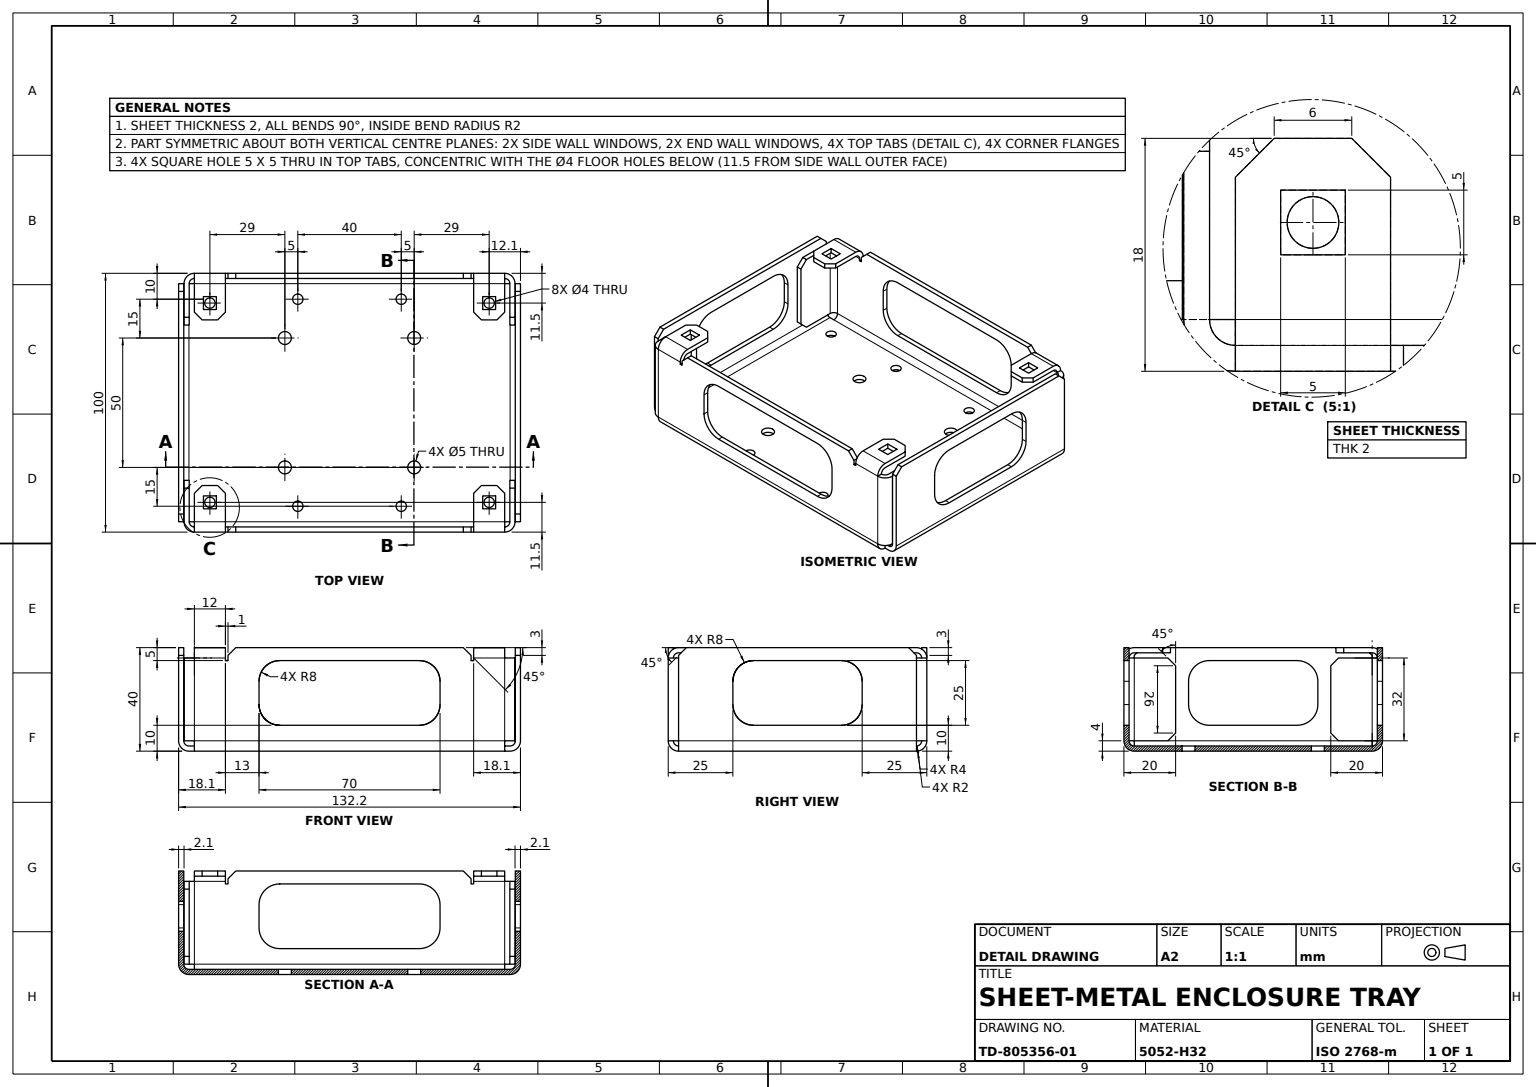
solid
v1 (51.5,38,-36)
v2 (56.5,38,-36)
e1 v1 v2 LINE
v3 (51.5,40,-36)
e2 v1 v3 LINE
v4 (56.5,40,-36)
e3 v3 v4 LINE
e4 v2 v4 LINE
face PLANE(AX(P(51.5,38,-36),D(0,0,1),D(0,-1,0))) rev [-e1 e2 e3 -e4]
v5 (54,0,36.5)
v6 (54,2,36.5)
e5 v5 v6 LINE
v7 (54,0,40.5)
e6 v5 v7 CIRCLE(AX(P(54,0,38.5),D(0,-1,0),D(0,0,-1)),2)
v8 (54,2,40.5)
e7 v7 v8 LINE
e8 v8 v6 CIRCLE(AX(P(54,2,38.5),D(0,1,0),D(0,0,1)),2)
face CYL(AX(P(54,-8,38.5),D(0,1,0),D(0,0,1)),2) rev [-e5 e6 e7 e8]
v9 (62,4,46)
v10 (64,4,46)
e9 v9 v10 LINE
v11 (60,4,50)
e10 v10 v11 CIRCLE(AX(P(60,4,46),D(0,-1,0),D(0,0,-1)),4)
v12 (60,4,48)
e11 v12 v11 LINE
e12 v9 v12 CIRCLE(AX(P(60,4,46),D(0,-1,0),D(0,0,-1)),2)
face PLANE(AX(P(60,4,46),D(0,1,0),D(0,0,1))) rev [e9 e10 -e11 -e12]
v13 (62.1,0,46)
v14 (60,0,46)
e13 v13 v14 LINE
v15 (62.1,2,46)
e14 v15 v13 LINE
v16 (60,2,46)
e15 v15 v16 LINE
e16 v16 v14 LINE
face PLANE(AX(P(62.1,2,46),D(0,0,-1),D(0,-1,0))) rev [-e13 -e14 e15 e16]
v17 (-62,4,46)
v18 (-62,36,46)
e17 v17 v18 LINE
v19 (-60,36,48)
e18 v18 v19 CIRCLE(AX(P(-60,36,46),D(0,1,0),D(0,0,1)),2)
v20 (-60,4,48)
e19 v20 v19 LINE
e20 v20 v17 CIRCLE(AX(P(-60,4,46),D(0,-1,0),D(0,0,1)),2)
face CYL(AX(P(-60,36,46),D(0,1,0),D(-1,0,0)),2) rev [e17 e18 -e19 e20]
v21 (-51,40,-32)
v22 (-48,40,-35)
e21 v21 v22 LINE
v23 (-51,38,-32)
e22 v23 v21 LINE
v24 (-48,38,-35)
e23 v24 v23 LINE
e24 v22 v24 LINE
face PLANE(AX(P(-48,40,-35),D(-0.707106781,0,-0.707106781),D(0,-1,0))) rev [-e21 -e22 -e23 -e24]
v25 (60,40,35)
v26 (57,40,32)
e25 v25 v26 LINE
v27 (60,38,35)
e26 v27 v25 LINE
v28 (57,38,32)
e27 v28 v27 LINE
e28 v26 v28 LINE
face PLANE(AX(P(57,40,32),D(-0.707106781,0,0.707106781),D(0,-1,0))) rev [-e25 -e26 -e27 -e28]
v29 (62.1,0,-46)
v30 (60,0,-46)
e29 v29 v30 LINE
v31 (60,2,-46)
e30 v31 v30 LINE
v32 (62.1,2,-46)
e31 v32 v31 LINE
e32 v32 v29 LINE
face PLANE(AX(P(62.1,2,-46),D(0,0,-1),D(0,-1,0))) [e29 -e30 -e31 e32]
v33 (-56.5,40,-36)
v34 (-51.5,40,-36)
e33 v33 v34 LINE
v35 (-51.5,38,-36)
e34 v35 v34 LINE
v36 (-56.5,38,-36)
e35 v36 v35 LINE
e36 v36 v33 LINE
face PLANE(AX(P(-51.5,38,-36),D(0,0,1),D(0,-1,0))) rev [e33 -e34 -e35 e36]
v37 (47,37,50)
v38 (44,40,50)
e37 v37 v38 LINE
v39 (47,37,48)
e38 v39 v37 LINE
v40 (44,40,48)
e39 v40 v39 LINE
e40 v38 v40 LINE
face PLANE(AX(P(47,37,48),D(-0.707106781,-0.707106781,0),D(0,0,1))) rev [-e37 -e38 -e39 -e40]
v41 (62,4,33)
e41 v9 v41 LINE
v42 (64,4,33)
e42 v41 v42 LINE
e43 v10 v42 LINE
face PLANE(AX(P(64,4,30),D(0,1,0),D(0,0,1))) rev [-e9 e41 e42 -e43]
v43 (-48,36,48)
e44 v43 v19 LINE
v44 (-60,38,46)
e45 v19 v44 CIRCLE(AX(P(-60,36,46),D(-1,0,0),D(0,0,-1)),2)
v45 (-48,38,46)
e46 v44 v45 LINE
e47 v45 v43 CIRCLE(AX(P(-48,36,46),D(1,0,0),D(0,0,-1)),2)
face CYL(AX(P(-48,36,46),D(1,0,0),D(0,1,0)),2) rev [e44 e45 e46 e47]
v46 (-47,37,50)
v47 (-47,37,48)
e48 v46 v47 LINE
v48 (-47,35,48)
e49 v47 v48 LINE
v49 (-47,35,50)
e50 v48 v49 LINE
e51 v49 v46 LINE
face PLANE(AX(P(-47,40,48),D(-1,0,0),D(0,0,1))) [e48 e49 e50 e51]
v50 (56.5,38,-41)
e52 v2 v50 LINE
v51 (51.5,38,-41)
e53 v50 v51 LINE
e54 v51 v1 LINE
v52 (48,38,-35)
v53 (48,38,-46)
e55 v52 v53 LINE
v54 (60,38,-46)
e56 v54 v53 LINE
v55 (60,38,-35)
e57 v54 v55 LINE
v56 (57,38,-32)
e58 v55 v56 LINE
v57 (51,38,-32)
e59 v56 v57 LINE
e60 v57 v52 LINE
face PLANE(AX(P(0,38,0),D(0,-1,0),D(0,0,-1))) [e52 e53 e54 e1] [e55 -e56 e57 e58 e59 e60]
v58 (60,4,-48)
e61 v31 v58 CIRCLE(AX(P(60,4,-46),D(1,0,0),D(0,0,1)),2)
v59 (60,4,-50)
e62 v30 v59 CIRCLE(AX(P(60,4,-46),D(1,0,0),D(0,0,1)),4)
e63 v58 v59 LINE
face PLANE(AX(P(60,4,-46),D(1,0,0),D(0,0,-1))) [-e61 e30 e62 -e63]
v60 (66.1,40,-43)
v61 (64.1,40,-43)
e64 v60 v61 LINE
v62 (66.1,37,-46)
e65 v62 v60 LINE
v63 (64.1,37,-46)
e66 v63 v62 LINE
e67 v61 v63 LINE
face PLANE(AX(P(66.1,40,-43),D(0,-0.707106781,0.707106781),D(-1,0,0))) rev [-e64 -e65 -e66 -e67]
v64 (-56.5,38,41)
v65 (-51.5,38,41)
e68 v64 v65 LINE
v66 (-56.5,40,41)
e69 v64 v66 LINE
v67 (-51.5,40,41)
e70 v66 v67 LINE
e71 v65 v67 LINE
face PLANE(AX(P(-51.5,38,41),D(0,0,1),D(0,-1,0))) rev [-e68 e69 e70 -e71]
v68 (-62,7,30)
v69 (-64,7,30)
e72 v68 v69 LINE
v70 (-62,4,33)
e73 v70 v68 LINE
v71 (-64,4,33)
e74 v71 v70 LINE
e75 v69 v71 LINE
face PLANE(AX(P(-64,4,33),D(0,0.707106781,0.707106781),D(1,0,0))) rev [-e72 -e73 -e74 -e75]
v72 (66.1,4,-46)
e76 v62 v72 LINE
v73 (64.1,4,-46)
e77 v73 v72 LINE
e78 v63 v73 LINE
face PLANE(AX(P(66.1,2,-46),D(0,0,-1),D(-1,0,0))) [e66 e76 -e77 -e78]
v74 (-57,38,32)
v75 (-51,38,32)
e79 v74 v75 LINE
v76 (-57,40,32)
e80 v74 v76 LINE
v77 (-51,40,32)
e81 v76 v77 LINE
e82 v77 v75 LINE
face PLANE(AX(P(-48,40,32),D(0,0,-1),D(0,1,0))) [-e79 e80 e81 e82]
v78 (-64,33,-30)
v79 (-64,36,-33)
e83 v78 v79 LINE
v80 (-64,36,-46)
e84 v79 v80 LINE
v81 (-64,4,-46)
e85 v81 v80 LINE
v82 (-64,4,-33)
e86 v81 v82 LINE
v83 (-64,7,-30)
e87 v82 v83 LINE
e88 v83 v78 LINE
face PLANE(AX(P(-64,0,0),D(1,0,0),D(0,0,-1))) rev [e83 e84 -e85 e86 e87 e88]
v84 (-54,0,36.5)
v85 (-54,0,40.5)
e89 v84 v85 CIRCLE(AX(P(-54,0,38.5),D(0,-1,0),D(0,0,-1)),2)
e90 v85 v84 CIRCLE(AX(P(-54,0,38.5),D(0,-1,0),D(0,0,-1)),2)
v86 (25,0,-27.5)
v87 (25,0,-22.5)
e91 v86 v87 CIRCLE(AX(P(25,0,-25),D(0,-1,0),D(0,0,-1)),2.5)
e92 v87 v86 CIRCLE(AX(P(25,0,-25),D(0,-1,0),D(0,0,-1)),2.5)
v88 (-25,0,-27.5)
v89 (-25,0,-22.5)
e93 v88 v89 CIRCLE(AX(P(-25,0,-25),D(0,-1,0),D(0,0,-1)),2.5)
e94 v89 v88 CIRCLE(AX(P(-25,0,-25),D(0,-1,0),D(0,0,-1)),2.5)
v90 (25,0,22.5)
v91 (25,0,27.5)
e95 v90 v91 CIRCLE(AX(P(25,0,25),D(0,-1,0),D(0,0,-1)),2.5)
e96 v91 v90 CIRCLE(AX(P(25,0,25),D(0,-1,0),D(0,0,-1)),2.5)
v92 (-25,0,22.5)
v93 (-25,0,27.5)
e97 v92 v93 CIRCLE(AX(P(-25,0,25),D(0,-1,0),D(0,0,-1)),2.5)
e98 v93 v92 CIRCLE(AX(P(-25,0,25),D(0,-1,0),D(0,0,-1)),2.5)
v94 (-20,0,38)
v95 (-20,0,42)
e99 v94 v95 CIRCLE(AX(P(-20,0,40),D(0,-1,0),D(0,0,-1)),2)
e100 v95 v94 CIRCLE(AX(P(-20,0,40),D(0,-1,0),D(0,0,-1)),2)
e101 v7 v5 CIRCLE(AX(P(54,0,38.5),D(0,-1,0),D(0,0,-1)),2)
v96 (-62.1,0,-46)
v97 (-60,0,-46)
e102 v96 v97 LINE
e103 v97 v30 LINE
e104 v29 v13 LINE
v98 (-60,0,46)
e105 v14 v98 LINE
v99 (-62.1,0,46)
e106 v99 v98 LINE
e107 v99 v96 LINE
v100 (-20,0,-38)
v101 (-20,0,-42)
e108 v100 v101 CIRCLE(AX(P(-20,0,-40),D(0,-1,0),D(0,0,-1)),2)
e109 v101 v100 CIRCLE(AX(P(-20,0,-40),D(0,-1,0),D(0,0,-1)),2)
v102 (20,0,38)
v103 (20,0,42)
e110 v102 v103 CIRCLE(AX(P(20,0,40),D(0,-1,0),D(0,0,-1)),2)
e111 v103 v102 CIRCLE(AX(P(20,0,40),D(0,-1,0),D(0,0,-1)),2)
v104 (-54,0,-36.5)
v105 (-54,0,-40.5)
e112 v104 v105 CIRCLE(AX(P(-54,0,-38.5),D(0,-1,0),D(0,0,-1)),2)
e113 v105 v104 CIRCLE(AX(P(-54,0,-38.5),D(0,-1,0),D(0,0,-1)),2)
v106 (54,0,-40.5)
v107 (54,0,-36.5)
e114 v106 v107 CIRCLE(AX(P(54,0,-38.5),D(0,-1,0),D(0,0,-1)),2)
e115 v107 v106 CIRCLE(AX(P(54,0,-38.5),D(0,-1,0),D(0,0,-1)),2)
v108 (20,0,-38)
v109 (20,0,-42)
e116 v108 v109 CIRCLE(AX(P(20,0,-40),D(0,-1,0),D(0,0,-1)),2)
e117 v109 v108 CIRCLE(AX(P(20,0,-40),D(0,-1,0),D(0,0,-1)),2)
face PLANE(AX(P(0,0,0),D(0,-1,0),D(0,0,-1))) [-e89 -e90] [-e91 -e92] [-e93 -e94] [-e95 -e96] [-e97 -e98] [-e99 -e100] [-e101 -e6] [e102 e103 -e29 e104 e13 e105 -e106 e107] [-e108 -e109] [-e110 -e111] [-e112 -e113] [-e114 -e115] [-e116 -e117]
v110 (-62,36,33)
e118 v18 v110 LINE
e119 v70 v17 LINE
v111 (-62,33,30)
e120 v111 v68 LINE
e121 v111 v110 LINE
face PLANE(AX(P(-62,0,0),D(1,0,0),D(0,0,-1))) [-e118 -e17 -e119 e73 -e120 e121]
v112 (-48,35,-48)
v113 (-47,35,-48)
e122 v112 v113 LINE
v114 (-47,35,-50)
e123 v113 v114 LINE
v115 (-48,35,-50)
e124 v114 v115 LINE
e125 v112 v115 LINE
face PLANE(AX(P(-48,35,-48),D(0,1,0),D(0,0,1))) [e122 e123 e124 -e125]
v116 (62,36,-46)
v117 (64,36,-46)
e126 v116 v117 LINE
v118 (60,36,-50)
e127 v117 v118 CIRCLE(AX(P(60,36,-46),D(0,1,0),D(0,0,1)),4)
v119 (60,36,-48)
e128 v119 v118 LINE
e129 v116 v119 CIRCLE(AX(P(60,36,-46),D(0,1,0),D(0,0,1)),2)
face PLANE(AX(P(60,36,-46),D(0,-1,0),D(0,0,-1))) rev [e126 e127 -e128 -e129]
v120 (-35,27,48)
v121 (-27,35,48)
e130 v120 v121 CIRCLE(AX(P(-27,27,48),D(0,0,-1),D(0,1,0)),8)
v122 (-27,35,50)
e131 v122 v121 LINE
v123 (-35,27,50)
e132 v123 v122 CIRCLE(AX(P(-27,27,50),D(0,0,-1),D(0,1,0)),8)
e133 v123 v120 LINE
face CYL(AX(P(-27,27,50),D(0,0,-1),D(0,1,0)),8) rev [e130 -e131 -e132 e133]
v124 (64,36,-33)
v125 (64,33,-30)
e134 v124 v125 LINE
v126 (64,7,-30)
e135 v125 v126 LINE
v127 (64,4,-33)
e136 v126 v127 LINE
v128 (64,4,-46)
e137 v127 v128 LINE
e138 v117 v128 LINE
e139 v117 v124 LINE
face PLANE(AX(P(64,0,0),D(-1,0,0),D(0,0,1))) rev [e134 e135 e136 e137 -e138 e139]
v129 (-51.5,38,-41)
v130 (-51.5,40,-41)
e140 v129 v130 LINE
e141 v35 v129 LINE
e142 v34 v130 LINE
face PLANE(AX(P(-51.5,38,-41),D(1,0,0),D(0,0,-1))) rev [-e140 -e141 e34 e142]
v131 (62,36,33)
v132 (62,33,30)
e143 v131 v132 LINE
v133 (64,36,33)
e144 v133 v131 LINE
v134 (64,33,30)
e145 v134 v133 LINE
e146 v132 v134 LINE
face PLANE(AX(P(64,36,33),D(0,-0.707106781,0.707106781),D(-1,0,0))) rev [-e143 -e144 -e145 -e146]
v135 (-64.1,37,-46)
v136 (-64.1,4,-46)
e147 v135 v136 LINE
v137 (-64.1,40,-43)
e148 v135 v137 LINE
v138 (-64.1,40,43)
e149 v138 v137 LINE
v139 (-64.1,37,46)
e150 v138 v139 LINE
v140 (-64.1,4,46)
e151 v140 v139 LINE
e152 v136 v140 LINE
v141 (-64.1,10,-17)
v142 (-64.1,18,-25)
e153 v141 v142 CIRCLE(AX(P(-64.1,18,-17),D(1,0,0),D(0,1,0)),8)
v143 (-64.1,10,17)
e154 v143 v141 LINE
v144 (-64.1,18,25)
e155 v144 v143 CIRCLE(AX(P(-64.1,18,17),D(1,0,0),D(0,1,0)),8)
v145 (-64.1,27,25)
e156 v145 v144 LINE
v146 (-64.1,35,17)
e157 v146 v145 CIRCLE(AX(P(-64.1,27,17),D(1,0,0),D(0,1,0)),8)
v147 (-64.1,35,-17)
e158 v147 v146 LINE
v148 (-64.1,27,-25)
e159 v148 v147 CIRCLE(AX(P(-64.1,27,-17),D(1,0,0),D(0,1,0)),8)
e160 v142 v148 LINE
face PLANE(AX(P(-64.1,0,0),D(1,0,0),D(0,1,0))) [-e147 e148 -e149 e150 -e151 -e152] [-e153 -e154 -e155 -e156 -e157 -e158 -e159 -e160]
v149 (48,35,-48)
v150 (48,35,-50)
e161 v149 v150 LINE
v151 (48,36,-48)
e162 v149 v151 LINE
v152 (48,36,-50)
e163 v151 v152 LINE
e164 v152 v150 LINE
face PLANE(AX(P(48,35,-48),D(-1,0,0),D(0,0,1))) [-e161 e162 e163 e164]
v153 (-48,36,50)
e165 v43 v153 LINE
v154 (-48,40,46)
e166 v45 v154 LINE
e167 v154 v153 CIRCLE(AX(P(-48,36,46),D(1,0,0),D(0,0,-1)),4)
face PLANE(AX(P(-48,36,46),D(-1,0,0),D(0,0,1))) rev [-e165 -e47 e166 e167]
v155 (64.1,4,46)
e168 v155 v73 LINE
e169 v73 v32 CIRCLE(AX(P(62.1,4,-46),D(0,0,-1),D(-1,0,0)),2)
e170 v32 v15 LINE
e171 v15 v155 CIRCLE(AX(P(62.1,4,46),D(0,0,1),D(-1,0,0)),2)
face CYL(AX(P(62.1,4,-46),D(0,0,-1),D(1,0,0)),2) rev [e168 e169 e170 e171]
v156 (-60,2,-46)
e172 v156 v31 LINE
v157 (-62.1,2,-46)
e173 v157 v156 LINE
v158 (-62.1,2,46)
e174 v158 v157 LINE
v159 (-60,2,46)
e175 v158 v159 LINE
e176 v16 v159 LINE
v160 (-54,2,-40.5)
v161 (-54,2,-36.5)
e177 v160 v161 CIRCLE(AX(P(-54,2,-38.5),D(0,1,0),D(0,0,1)),2)
e178 v161 v160 CIRCLE(AX(P(-54,2,-38.5),D(0,1,0),D(0,0,1)),2)
v162 (25,2,22.5)
v163 (25,2,27.5)
e179 v162 v163 CIRCLE(AX(P(25,2,25),D(0,1,0),D(0,0,-1)),2.5)
e180 v163 v162 CIRCLE(AX(P(25,2,25),D(0,1,0),D(0,0,-1)),2.5)
v164 (-20,2,42)
v165 (-20,2,38)
e181 v164 v165 CIRCLE(AX(P(-20,2,40),D(0,1,0),D(0,0,-1)),2)
e182 v165 v164 CIRCLE(AX(P(-20,2,40),D(0,1,0),D(0,0,-1)),2)
e183 v6 v8 CIRCLE(AX(P(54,2,38.5),D(0,1,0),D(0,0,1)),2)
v166 (-25,2,22.5)
v167 (-25,2,27.5)
e184 v166 v167 CIRCLE(AX(P(-25,2,25),D(0,1,0),D(0,0,1)),2.5)
e185 v167 v166 CIRCLE(AX(P(-25,2,25),D(0,1,0),D(0,0,1)),2.5)
v168 (-54,2,40.5)
v169 (-54,2,36.5)
e186 v168 v169 CIRCLE(AX(P(-54,2,38.5),D(0,1,0),D(0,0,-1)),2)
e187 v169 v168 CIRCLE(AX(P(-54,2,38.5),D(0,1,0),D(0,0,-1)),2)
v170 (20,2,38)
v171 (20,2,42)
e188 v170 v171 CIRCLE(AX(P(20,2,40),D(0,1,0),D(0,0,-1)),2)
e189 v171 v170 CIRCLE(AX(P(20,2,40),D(0,1,0),D(0,0,-1)),2)
v172 (54,2,-40.5)
v173 (54,2,-36.5)
e190 v172 v173 CIRCLE(AX(P(54,2,-38.5),D(0,1,0),D(0,0,-1)),2)
e191 v173 v172 CIRCLE(AX(P(54,2,-38.5),D(0,1,0),D(0,0,-1)),2)
v174 (25,2,-22.5)
v175 (25,2,-27.5)
e192 v174 v175 CIRCLE(AX(P(25,2,-25),D(0,1,0),D(0,0,1)),2.5)
e193 v175 v174 CIRCLE(AX(P(25,2,-25),D(0,1,0),D(0,0,1)),2.5)
v176 (20,2,-42)
v177 (20,2,-38)
e194 v176 v177 CIRCLE(AX(P(20,2,-40),D(0,1,0),D(0,0,1)),2)
e195 v177 v176 CIRCLE(AX(P(20,2,-40),D(0,1,0),D(0,0,1)),2)
v178 (-25,2,-27.5)
v179 (-25,2,-22.5)
e196 v178 v179 CIRCLE(AX(P(-25,2,-25),D(0,1,0),D(0,0,-1)),2.5)
e197 v179 v178 CIRCLE(AX(P(-25,2,-25),D(0,1,0),D(0,0,-1)),2.5)
v180 (-20,2,-42)
v181 (-20,2,-38)
e198 v180 v181 CIRCLE(AX(P(-20,2,-40),D(0,1,0),D(0,0,1)),2)
e199 v181 v180 CIRCLE(AX(P(-20,2,-40),D(0,1,0),D(0,0,1)),2)
face PLANE(AX(P(0,2,0),D(0,-1,0),D(0,0,-1))) rev [-e172 -e173 -e174 e175 -e176 -e15 -e170 e31] [-e177 -e178] [-e179 -e180] [-e181 -e182] [-e8 -e183] [-e184 -e185] [-e186 -e187] [-e188 -e189] [-e190 -e191] [-e192 -e193] [-e194 -e195] [-e196 -e197] [-e198 -e199]
v182 (48,40,-46)
e200 v53 v182 LINE
v183 (48,40,-35)
e201 v52 v183 LINE
e202 v183 v182 LINE
face PLANE(AX(P(48,40,-48),D(-1,0,0),D(0,0,1))) [-e200 -e55 e201 e202]
v184 (-60,36,50)
e203 v19 v184 LINE
v185 (-64,36,46)
e204 v18 v185 LINE
e205 v185 v184 CIRCLE(AX(P(-60,36,46),D(0,1,0),D(0,0,1)),4)
face PLANE(AX(P(-60,36,46),D(0,-1,0),D(0,0,-1))) rev [-e203 -e18 e204 e205]
e206 v105 v160 LINE
e207 v104 v161 LINE
face CYL(AX(P(-54,-8,-38.5),D(0,1,0),D(0,0,1)),2) rev [e112 e206 e177 -e207]
v186 (-60,40,46)
e208 v44 v186 LINE
e209 v184 v186 CIRCLE(AX(P(-60,36,46),D(-1,0,0),D(0,0,-1)),4)
face PLANE(AX(P(-60,36,46),D(-1,0,0),D(0,0,1))) [-e208 -e45 e203 e209]
v187 (44,40,-48)
v188 (44,40,-50)
e210 v187 v188 LINE
v189 (47,37,-48)
e211 v189 v187 LINE
v190 (47,37,-50)
e212 v190 v189 LINE
e213 v188 v190 LINE
face PLANE(AX(P(44,40,-50),D(0.707106781,0.707106781,0),D(0,0,1))) [-e210 -e211 -e212 -e213]
v191 (-62,36,-46)
v192 (-62,4,-46)
e214 v191 v192 LINE
v193 (-60,4,-48)
e215 v192 v193 CIRCLE(AX(P(-60,4,-46),D(0,-1,0),D(0,0,-1)),2)
v194 (-60,36,-48)
e216 v193 v194 LINE
e217 v194 v191 CIRCLE(AX(P(-60,36,-46),D(0,1,0),D(0,0,-1)),2)
face CYL(AX(P(-60,4,-46),D(0,-1,0),D(-1,0,0)),2) rev [e214 e215 e216 e217]
v195 (64.1,27,25)
v196 (66.1,27,25)
e218 v195 v196 LINE
v197 (64.1,35,17)
e219 v195 v197 CIRCLE(AX(P(64.1,27,17),D(-1,0,0),D(0,-1,0)),8)
v198 (66.1,35,17)
e220 v197 v198 LINE
e221 v198 v196 CIRCLE(AX(P(66.1,27,17),D(1,0,0),D(0,1,0)),8)
face CYL(AX(P(-66.1,27,17),D(1,0,0),D(0,1,0)),8) rev [-e218 e219 e220 e221]
v199 (-64,33,30)
e222 v199 v111 LINE
v200 (-64,36,33)
e223 v200 v199 LINE
e224 v110 v200 LINE
face PLANE(AX(P(-64,33,30),D(0,-0.707106781,0.707106781),D(1,0,0))) rev [-e121 -e222 -e223 -e224]
v201 (27,10,50)
v202 (-27,10,50)
e225 v201 v202 LINE
v203 (27,10,48)
e226 v201 v203 LINE
v204 (-27,10,48)
e227 v203 v204 LINE
e228 v202 v204 LINE
face PLANE(AX(P(27,10,50),D(0,-1,0),D(0,0,-1))) rev [-e225 e226 e227 -e228]
v205 (62,7,30)
e229 v205 v41 LINE
v206 (64,7,30)
e230 v206 v205 LINE
e231 v42 v206 LINE
face PLANE(AX(P(64,7,30),D(0,0.707106781,0.707106781),D(-1,0,0))) rev [-e229 -e230 -e231 -e42]
v207 (62,36,46)
e232 v207 v9 LINE
e233 v131 v207 LINE
e234 v205 v132 LINE
face PLANE(AX(P(62,0,0),D(-1,0,0),D(0,0,1))) [-e232 -e233 e143 -e234 e229 -e41]
v208 (-60,38,-35)
v209 (-60,40,-35)
e235 v208 v209 LINE
v210 (-60,40,-46)
e236 v210 v209 LINE
v211 (-60,38,-46)
e237 v211 v210 LINE
e238 v211 v208 LINE
face PLANE(AX(P(-60,40,-32),D(1,0,0),D(0,0,-1))) rev [e235 -e236 -e237 e238]
v212 (35,18,50)
e239 v212 v201 CIRCLE(AX(P(27,18,50),D(0,0,-1),D(0,1,0)),8)
v213 (35,18,48)
e240 v212 v213 LINE
e241 v213 v203 CIRCLE(AX(P(27,18,48),D(0,0,-1),D(0,1,0)),8)
face CYL(AX(P(27,18,50),D(0,0,-1),D(0,1,0)),8) rev [-e226 -e239 e240 e241]
v214 (-66.1,10,17)
e242 v214 v143 LINE
v215 (-66.1,18,25)
e243 v215 v214 CIRCLE(AX(P(-66.1,18,17),D(1,0,0),D(0,-1,0)),8)
e244 v215 v144 LINE
face CYL(AX(P(-66.1,18,17),D(1,0,0),D(0,1,0)),8) rev [-e242 -e243 e244 e155]
v216 (66.1,40,43)
v217 (66.1,37,46)
e245 v216 v217 LINE
v218 (64.1,40,43)
e246 v218 v216 LINE
v219 (64.1,37,46)
e247 v219 v218 LINE
e248 v217 v219 LINE
face PLANE(AX(P(66.1,37,46),D(0,-0.707106781,-0.707106781),D(-1,0,0))) rev [-e245 -e246 -e247 -e248]
v220 (-35,18,-50)
v221 (-35,27,-50)
e249 v220 v221 LINE
v222 (-27,10,-50)
e250 v222 v220 CIRCLE(AX(P(-27,18,-50),D(0,0,-1),D(0,1,0)),8)
v223 (27,10,-50)
e251 v223 v222 LINE
v224 (35,18,-50)
e252 v224 v223 CIRCLE(AX(P(27,18,-50),D(0,0,-1),D(0,1,0)),8)
v225 (35,27,-50)
e253 v225 v224 LINE
v226 (27,35,-50)
e254 v226 v225 CIRCLE(AX(P(27,27,-50),D(0,0,-1),D(0,1,0)),8)
v227 (-27,35,-50)
e255 v227 v226 LINE
e256 v221 v227 CIRCLE(AX(P(-27,27,-50),D(0,0,-1),D(0,1,0)),8)
v228 (-60,4,-50)
e257 v228 v59 LINE
v229 (-60,36,-50)
e258 v228 v229 LINE
v230 (-48,36,-50)
e259 v229 v230 LINE
e260 v115 v230 LINE
v231 (-47,37,-50)
e261 v231 v114 LINE
v232 (-44,40,-50)
e262 v231 v232 LINE
e263 v232 v188 LINE
v233 (47,35,-50)
e264 v233 v190 LINE
e265 v150 v233 LINE
e266 v152 v118 LINE
e267 v118 v59 LINE
face PLANE(AX(P(0,0,-50),D(0,0,1),D(0,-1,0))) rev [-e249 -e250 -e251 -e252 -e253 -e254 -e255 -e256] [-e257 e258 e259 -e260 -e124 -e261 e262 e263 e213 -e264 -e265 -e164 e266 e267]
v234 (-48,38,35)
v235 (-48,40,35)
e268 v234 v235 LINE
e269 v75 v234 LINE
e270 v235 v77 LINE
face PLANE(AX(P(-51,40,32),D(-0.707106781,0,0.707106781),D(0,-1,0))) rev [-e268 -e269 -e82 -e270]
v236 (-48,36,-48)
e271 v236 v230 LINE
e272 v236 v112 LINE
face PLANE(AX(P(-48,36,-48),D(1,0,0),D(0,0,-1))) [e125 e260 -e271 e272]
v237 (-51.5,38,36)
v238 (-51.5,40,36)
e273 v237 v238 LINE
e274 v65 v237 LINE
e275 v67 v238 LINE
face PLANE(AX(P(-51.5,38,41),D(1,0,0),D(0,0,-1))) rev [-e273 -e274 e71 e275]
v239 (-48,35,50)
e276 v153 v239 LINE
v240 (-48,35,48)
e277 v240 v239 LINE
e278 v240 v43 LINE
face PLANE(AX(P(-48,35,48),D(1,0,0),D(0,0,-1))) [e276 -e277 e278 e165]
e279 v109 v176 LINE
e280 v108 v177 LINE
face CYL(AX(P(20,-8,-40),D(0,1,0),D(0,0,1)),2) rev [e279 e194 -e280 e116]
e281 v155 v219 LINE
e282 v218 v61 LINE
v241 (64.1,27,-25)
v242 (64.1,18,-25)
e283 v241 v242 LINE
v243 (64.1,35,-17)
e284 v243 v241 CIRCLE(AX(P(64.1,27,-17),D(-1,0,0),D(0,-1,0)),8)
e285 v197 v243 LINE
v244 (64.1,18,25)
e286 v244 v195 LINE
v245 (64.1,10,17)
e287 v245 v244 CIRCLE(AX(P(64.1,18,17),D(-1,0,0),D(0,-1,0)),8)
v246 (64.1,10,-17)
e288 v246 v245 LINE
e289 v242 v246 CIRCLE(AX(P(64.1,18,-17),D(-1,0,0),D(0,-1,0)),8)
face PLANE(AX(P(64.1,0,0),D(-1,0,0),D(0,1,0))) [e67 e78 -e168 e281 e247 e282] [-e283 -e284 -e285 -e219 -e286 -e287 -e288 -e289]
v247 (-62,36,-33)
e290 v247 v191 LINE
v248 (-62,33,-30)
e291 v247 v248 LINE
v249 (-62,7,-30)
e292 v249 v248 LINE
v250 (-62,4,-33)
e293 v249 v250 LINE
e294 v192 v250 LINE
face PLANE(AX(P(-62,0,0),D(1,0,0),D(0,0,-1))) [-e214 -e290 e291 -e292 e293 -e294]
v251 (-64,4,46)
e295 v17 v251 LINE
e296 v71 v251 LINE
face PLANE(AX(P(-64,4,48),D(0,1,0),D(0,0,1))) rev [e74 e119 e295 -e296]
e297 v153 v184 LINE
e298 v154 v186 LINE
face CYL(AX(P(-48,36,46),D(1,0,0),D(0,1,0)),4) [-e209 -e297 -e167 e298]
e299 v185 v251 LINE
e300 v185 v200 LINE
e301 v199 v69 LINE
face PLANE(AX(P(-64,0,0),D(1,0,0),D(0,0,-1))) rev [-e299 e300 e223 e301 e75 e296]
e302 v206 v134 LINE
face PLANE(AX(P(64,36,30),D(0,0,1),D(1,0,0))) rev [e230 e234 e146 -e302]
e303 v89 v179 LINE
e304 v88 v178 LINE
face CYL(AX(P(-25,-8,-25),D(0,1,0),D(0,0,1)),2.5) rev [e196 -e303 e94 e304]
e305 v90 v162 LINE
e306 v91 v163 LINE
face CYL(AX(P(25,-8,25),D(0,1,0),D(0,0,1)),2.5) rev [e96 e305 e179 -e306]
v252 (51.5,38,36)
v253 (51.5,38,41)
e307 v252 v253 LINE
v254 (51.5,40,36)
e308 v252 v254 LINE
v255 (51.5,40,41)
e309 v254 v255 LINE
e310 v253 v255 LINE
face PLANE(AX(P(51.5,38,41),D(-1,0,0),D(0,0,1))) rev [-e307 e308 e309 -e310]
v256 (62,36,-33)
e311 v116 v256 LINE
e312 v256 v124 LINE
face PLANE(AX(P(64,36,-30),D(0,-1,0),D(0,0,-1))) rev [-e126 e311 e312 -e139]
v257 (-48,38,-46)
v258 (-48,40,-46)
e313 v257 v258 LINE
e314 v22 v258 LINE
e315 v24 v257 LINE
face PLANE(AX(P(-48,40,-48),D(-1,0,0),D(0,0,1))) rev [e313 -e314 e24 e315]
v259 (-66.1,40,-43)
v260 (-66.1,37,-46)
e316 v259 v260 LINE
e317 v137 v259 LINE
e318 v260 v135 LINE
face PLANE(AX(P(-66.1,37,-46),D(0,-0.707106781,0.707106781),D(1,0,0))) rev [-e316 -e317 -e148 -e318]
e319 v100 v181 LINE
e320 v101 v180 LINE
face CYL(AX(P(-20,-8,-40),D(0,1,0),D(0,0,1)),2) rev [e319 e199 -e320 e109]
e321 v94 v165 LINE
e322 v95 v164 LINE
face CYL(AX(P(-20,-8,40),D(0,1,0),D(0,0,1)),2) rev [-e321 e99 e322 e181]
v261 (-47,37,-48)
e323 v113 v261 LINE
e324 v261 v231 LINE
face PLANE(AX(P(-47,35,-48),D(-1,0,0),D(0,0,1))) [e323 e324 e261 -e123]
v262 (57,40,-32)
e325 v56 v262 LINE
v263 (51,40,-32)
e326 v262 v263 LINE
e327 v263 v57 LINE
face PLANE(AX(P(48,40,-32),D(0,0,1),D(0,-1,0))) [e325 e326 e327 -e59]
v264 (35,18,-48)
v265 (35,27,-48)
e328 v264 v265 LINE
e329 v265 v225 LINE
e330 v264 v224 LINE
face PLANE(AX(P(35,18,50),D(1,0,0),D(0,0,-1))) rev [e328 e329 e253 -e330]
e331 v72 v29 CIRCLE(AX(P(62.1,4,-46),D(0,0,-1),D(-1,0,0)),4)
face PLANE(AX(P(62.1,4,-46),D(0,0,1),D(1,0,0))) rev [e77 e331 -e32 -e169]
v266 (56.5,38,36)
e332 v266 v252 LINE
v267 (56.5,40,36)
e333 v266 v267 LINE
e334 v267 v254 LINE
face PLANE(AX(P(51.5,38,36),D(0,0,-1),D(0,1,0))) rev [-e308 -e332 e333 e334]
v268 (47,35,-48)
e335 v268 v233 LINE
e336 v268 v149 LINE
face PLANE(AX(P(47,35,-48),D(0,1,0),D(0,0,1))) [e161 e265 -e335 e336]
v269 (27,10,-48)
e337 v269 v223 LINE
e338 v269 v264 CIRCLE(AX(P(27,18,-48),D(0,0,1),D(0,-1,0)),8)
face CYL(AX(P(27,18,50),D(0,0,-1),D(0,1,0)),8) rev [e330 e252 -e337 e338]
v270 (-57,40,-32)
e339 v270 v21 LINE
v271 (-57,38,-32)
e340 v270 v271 LINE
e341 v271 v23 LINE
face PLANE(AX(P(-48,40,-32),D(0,0,-1),D(0,1,0))) rev [e22 -e339 e340 e341]
v272 (60,40,46)
e342 v272 v25 LINE
v273 (60,38,46)
e343 v273 v272 LINE
e344 v273 v27 LINE
face PLANE(AX(P(60,40,32),D(-1,0,0),D(0,0,1))) rev [e26 -e342 -e343 e344]
v274 (-66.1,4,46)
e345 v274 v99 CIRCLE(AX(P(-62.1,4,46),D(0,0,1),D(1,0,0)),4)
v275 (-66.1,4,-46)
e346 v274 v275 LINE
e347 v96 v275 CIRCLE(AX(P(-62.1,4,-46),D(0,0,-1),D(1,0,0)),4)
face CYL(AX(P(-62.1,4,46),D(0,0,1),D(-1,0,0)),4) [-e107 -e345 e346 -e347]
v276 (-35,18,-48)
e348 v276 v220 LINE
v277 (-27,10,-48)
e349 v276 v277 CIRCLE(AX(P(-27,18,-48),D(0,0,1),D(0,-1,0)),8)
e350 v277 v222 LINE
face CYL(AX(P(-27,18,50),D(0,0,-1),D(0,1,0)),8) rev [-e348 e349 e350 e250]
e351 v228 v97 CIRCLE(AX(P(-60,4,-46),D(-1,0,0),D(0,0,1)),4)
face CYL(AX(P(-60,4,-46),D(-1,0,0),D(0,0,-1)),4) [e257 -e62 -e103 -e351]
e352 v81 v228 CIRCLE(AX(P(-60,4,-46),D(0,-1,0),D(0,0,-1)),4)
e353 v229 v80 CIRCLE(AX(P(-60,36,-46),D(0,1,0),D(0,0,-1)),4)
face CYL(AX(P(-60,4,-46),D(0,-1,0),D(-1,0,0)),4) [-e258 -e352 e85 -e353]
v278 (35,27,48)
e354 v278 v213 LINE
v279 (35,27,50)
e355 v279 v212 LINE
e356 v279 v278 LINE
face PLANE(AX(P(35,18,50),D(1,0,0),D(0,0,-1))) rev [e354 -e240 -e355 e356]
v280 (62,4,-46)
e357 v280 v116 LINE
v281 (62,4,-33)
e358 v281 v280 LINE
v282 (62,7,-30)
e359 v281 v282 LINE
v283 (62,33,-30)
e360 v283 v282 LINE
e361 v283 v256 LINE
face PLANE(AX(P(62,0,0),D(-1,0,0),D(0,0,1))) [-e311 -e357 -e358 e359 -e360 e361]
face CYL(AX(P(-20,-8,-40),D(0,1,0),D(0,0,1)),2) rev [-e319 e108 e320 e198]
v284 (51.5,40,-41)
e362 v51 v284 LINE
e363 v284 v3 LINE
face PLANE(AX(P(51.5,38,-41),D(-1,0,0),D(0,0,1))) rev [-e54 e362 e363 -e2]
v285 (-56.5,38,36)
e364 v285 v64 LINE
v286 (-56.5,40,36)
e365 v285 v286 LINE
e366 v286 v66 LINE
face PLANE(AX(P(-56.5,38,41),D(-1,0,0),D(0,0,1))) rev [-e364 e365 e366 -e69]
e367 v85 v168 LINE
e368 v84 v169 LINE
face CYL(AX(P(-54,-8,38.5),D(0,1,0),D(0,0,1)),2) rev [e89 e367 e186 -e368]
e369 v250 v82 LINE
e370 v83 v249 LINE
face PLANE(AX(P(-64,7,-30),D(0,0.707106781,-0.707106781),D(1,0,0))) rev [-e87 -e369 -e293 -e370]
e371 v209 v270 LINE
e372 v271 v208 LINE
face PLANE(AX(P(-57,40,-32),D(0.707106781,0,-0.707106781),D(0,-1,0))) rev [-e340 -e371 -e235 -e372]
e373 v53 v151 CIRCLE(AX(P(48,36,-46),D(-1,0,0),D(0,0,1)),2)
e374 v182 v152 CIRCLE(AX(P(48,36,-46),D(-1,0,0),D(0,0,1)),4)
face PLANE(AX(P(48,36,-46),D(1,0,0),D(0,0,-1))) rev [-e163 -e373 e200 e374]
e375 v58 v193 LINE
e376 v193 v156 CIRCLE(AX(P(-60,4,-46),D(-1,0,0),D(0,0,1)),2)
face CYL(AX(P(-60,4,-46),D(-1,0,0),D(0,0,-1)),2) rev [e61 e375 e376 e172]
v287 (-66.1,37,46)
e377 v274 v287 LINE
v288 (-66.1,40,43)
e378 v287 v288 LINE
e379 v288 v259 LINE
e380 v260 v275 LINE
v289 (-66.1,18,-25)
v290 (-66.1,27,-25)
e381 v289 v290 LINE
v291 (-66.1,35,-17)
e382 v290 v291 CIRCLE(AX(P(-66.1,27,-17),D(1,0,0),D(0,1,0)),8)
v292 (-66.1,35,17)
e383 v291 v292 LINE
v293 (-66.1,27,25)
e384 v292 v293 CIRCLE(AX(P(-66.1,27,17),D(1,0,0),D(0,1,0)),8)
e385 v293 v215 LINE
v294 (-66.1,10,-17)
e386 v214 v294 LINE
e387 v294 v289 CIRCLE(AX(P(-66.1,18,-17),D(1,0,0),D(0,1,0)),8)
face PLANE(AX(P(-66.1,0,0),D(1,0,0),D(0,1,0))) rev [e377 e378 e379 e316 e380 -e346] [e381 e382 e383 e384 e385 e243 e386 e387]
e388 v125 v283 LINE
face PLANE(AX(P(64,33,-30),D(0,-0.707106781,-0.707106781),D(-1,0,0))) rev [-e312 -e361 -e388 -e134]
e389 v291 v147 LINE
e390 v290 v148 LINE
face CYL(AX(P(-66.1,27,-17),D(1,0,0),D(0,1,0)),8) rev [e159 -e389 -e382 e390]
face PLANE(AX(P(-64,4,30),D(0,0,1),D(1,0,0))) rev [e120 e72 -e301 e222]
v295 (66.1,4,46)
e391 v155 v295 LINE
e392 v295 v217 LINE
face PLANE(AX(P(66.1,40,46),D(0,0,1),D(1,0,0))) [e391 e392 e248 -e281]
e393 v72 v295 LINE
e394 v13 v295 CIRCLE(AX(P(62.1,4,46),D(0,0,1),D(-1,0,0)),4)
face CYL(AX(P(62.1,4,-46),D(0,0,-1),D(1,0,0)),4) [-e331 e393 -e394 -e104]
e395 v159 v98 LINE
e396 v158 v99 LINE
face PLANE(AX(P(-62.1,2,46),D(0,0,1),D(0,-1,0))) [-e395 -e175 e396 e106]
e397 v139 v287 LINE
e398 v288 v138 LINE
face PLANE(AX(P(-66.1,40,43),D(0,-0.707106781,-0.707106781),D(1,0,0))) rev [-e378 -e397 -e150 -e398]
v296 (-35,18,48)
e399 v296 v120 LINE
e400 v204 v296 CIRCLE(AX(P(-27,18,48),D(0,0,-1),D(0,1,0)),8)
v297 (27,35,48)
e401 v297 v278 CIRCLE(AX(P(27,27,48),D(0,0,-1),D(0,1,0)),8)
e402 v121 v297 LINE
v298 (47,35,48)
e403 v298 v39 LINE
v299 (48,35,48)
e404 v299 v298 LINE
v300 (48,36,48)
e405 v300 v299 LINE
v301 (60,36,48)
e406 v301 v300 LINE
e407 v301 v12 LINE
e408 v20 v12 LINE
e409 v48 v240 LINE
v302 (-44,40,48)
e410 v47 v302 LINE
e411 v302 v40 LINE
face PLANE(AX(P(0,0,48),D(0,0,-1),D(0,-1,0))) [-e130 -e399 -e400 -e227 -e241 -e354 -e401 -e402] [e39 -e403 -e404 -e405 -e406 e407 -e408 e19 -e44 -e278 -e409 -e49 e410 e411]
e412 v191 v80 LINE
e413 v79 v247 LINE
face PLANE(AX(P(-64,36,-48),D(0,-1,0),D(0,0,-1))) rev [e290 e412 -e84 e413]
v303 (47,35,50)
e414 v298 v303 LINE
v304 (48,35,50)
e415 v303 v304 LINE
e416 v299 v304 LINE
face PLANE(AX(P(48,35,48),D(0,1,0),D(0,0,1))) [e404 e414 e415 -e416]
e417 v248 v78 LINE
face PLANE(AX(P(-64,36,-30),D(0,0,-1),D(-1,0,0))) rev [e417 -e88 e370 e292]
e418 v11 v14 CIRCLE(AX(P(60,4,46),D(1,0,0),D(0,0,-1)),4)
v305 (-60,4,50)
e419 v11 v305 LINE
e420 v98 v305 CIRCLE(AX(P(-60,4,46),D(-1,0,0),D(0,0,-1)),4)
face CYL(AX(P(60,4,46),D(1,0,0),D(0,0,1)),4) [-e105 -e418 e419 -e420]
v306 (-27,35,-48)
e421 v306 v227 LINE
v307 (-35,27,-48)
e422 v306 v307 CIRCLE(AX(P(-27,27,-48),D(0,0,1),D(0,-1,0)),8)
e423 v307 v221 LINE
face CYL(AX(P(-27,27,50),D(0,0,-1),D(0,1,0)),8) rev [e256 -e421 e422 e423]
e424 v183 v263 LINE
face PLANE(AX(P(51,40,-32),D(0.707106781,0,-0.707106781),D(0,-1,0))) rev [-e327 -e424 -e201 -e60]
e425 v106 v172 LINE
e426 v107 v173 LINE
face CYL(AX(P(54,-8,-38.5),D(0,1,0),D(0,0,1)),2) rev [e425 e190 -e426 e115]
e427 v59 v128 CIRCLE(AX(P(60,4,-46),D(0,-1,0),D(0,0,1)),4)
e428 v280 v128 LINE
e429 v58 v280 CIRCLE(AX(P(60,4,-46),D(0,-1,0),D(0,0,1)),2)
face PLANE(AX(P(60,4,-46),D(0,-1,0),D(0,0,-1))) [e63 e427 -e428 -e429]
e430 v12 v16 CIRCLE(AX(P(60,4,46),D(1,0,0),D(0,0,-1)),2)
face PLANE(AX(P(60,4,46),D(-1,0,0),D(0,0,1))) rev [e418 -e16 -e430 e11]
e431 v277 v269 LINE
face PLANE(AX(P(27,10,50),D(0,-1,0),D(0,0,-1))) rev [e251 -e350 e431 e337]
v308 (48,40,35)
v309 (48,38,35)
e432 v308 v309 LINE
v310 (51,40,32)
e433 v310 v308 LINE
v311 (51,38,32)
e434 v311 v310 LINE
e435 v309 v311 LINE
face PLANE(AX(P(48,40,35),D(0.707106781,0,0.707106781),D(0,-1,0))) rev [-e432 -e433 -e434 -e435]
e436 v230 v258 CIRCLE(AX(P(-48,36,-46),D(1,0,0),D(0,0,1)),4)
e437 v236 v257 CIRCLE(AX(P(-48,36,-46),D(1,0,0),D(0,0,1)),2)
face PLANE(AX(P(-48,36,-46),D(1,0,0),D(0,0,-1))) [e271 e436 -e313 -e437]
face CYL(AX(P(54,-8,-38.5),D(0,1,0),D(0,0,1)),2) rev [e426 e191 -e425 e114]
v312 (56.5,40,-41)
e438 v50 v312 LINE
e439 v312 v284 LINE
face PLANE(AX(P(51.5,38,-41),D(0,0,-1),D(0,1,0))) rev [-e53 e438 e439 -e362]
e440 v156 v97 LINE
e441 v193 v228 LINE
face PLANE(AX(P(-60,4,-46),D(1,0,0),D(0,0,-1))) rev [-e440 -e376 e441 e351]
face PLANE(AX(P(-64,36,30),D(0,-1,0),D(0,0,-1))) rev [e118 e224 -e300 -e204]
v313 (60,36,50)
v314 (64,36,46)
e442 v313 v314 CIRCLE(AX(P(60,36,46),D(0,1,0),D(0,0,-1)),4)
e443 v313 v11 LINE
e444 v10 v314 LINE
face CYL(AX(P(60,4,46),D(0,-1,0),D(1,0,0)),4) [-e442 e443 -e10 e444]
e445 v20 v305 LINE
e446 v305 v251 CIRCLE(AX(P(-60,4,46),D(0,-1,0),D(0,0,1)),4)
face PLANE(AX(P(-60,4,46),D(0,-1,0),D(0,0,-1))) [e445 e446 -e295 -e20]
face PLANE(AX(P(62.1,4,46),D(0,0,1),D(1,0,0))) [-e171 e14 e394 -e391]
v315 (66.1,18,25)
e447 v196 v315 LINE
e448 v244 v315 LINE
face PLANE(AX(P(-66.1,18,25),D(0,0,1),D(1,0,0))) rev [e218 e447 -e448 e286]
v316 (66.1,27,-25)
e449 v241 v316 LINE
v317 (66.1,18,-25)
e450 v242 v317 LINE
e451 v317 v316 LINE
face PLANE(AX(P(-66.1,18,-25),D(0,0,-1),D(-1,0,0))) rev [-e449 e283 e450 e451]
v318 (60,40,-35)
e452 v318 v55 LINE
e453 v262 v318 LINE
face PLANE(AX(P(60,40,-35),D(-0.707106781,0,-0.707106781),D(0,-1,0))) rev [-e452 -e453 -e325 -e58]
v319 (-60,38,35)
e454 v44 v319 LINE
v320 (-60,40,35)
e455 v186 v320 LINE
e456 v320 v319 LINE
face PLANE(AX(P(-60,40,32),D(-1,0,0),D(0,0,1))) [-e454 e208 e455 e456]
e457 v292 v146 LINE
e458 v293 v145 LINE
face CYL(AX(P(-66.1,27,17),D(1,0,0),D(0,1,0)),8) rev [-e384 e457 e157 -e458]
v321 (-44,40,50)
e459 v321 v46 LINE
e460 v302 v321 LINE
face PLANE(AX(P(-44,40,50),D(0.707106781,-0.707106781,0),D(0,0,1))) rev [-e48 -e459 -e460 -e410]
v322 (-44,40,-48)
e461 v322 v261 LINE
e462 v232 v322 LINE
face PLANE(AX(P(-47,37,-48),D(-0.707106781,0.707106781,0),D(0,0,1))) [-e324 -e461 -e462 -e262]
v323 (60,40,-46)
e463 v54 v323 LINE
e464 v323 v318 LINE
face PLANE(AX(P(60,40,-32),D(1,0,0),D(0,0,-1))) [e463 e464 e452 -e57]
e465 v93 v167 LINE
e466 v92 v166 LINE
face CYL(AX(P(-25,-8,25),D(0,1,0),D(0,0,1)),2.5) rev [e97 e465 e185 -e466]
e467 v272 v313 CIRCLE(AX(P(60,36,46),D(1,0,0),D(0,0,-1)),4)
e468 v301 v313 LINE
e469 v273 v301 CIRCLE(AX(P(60,36,46),D(1,0,0),D(0,0,-1)),2)
face PLANE(AX(P(60,36,46),D(-1,0,0),D(0,0,1))) rev [e467 -e468 -e469 e343]
e470 v87 v174 LINE
e471 v86 v175 LINE
face CYL(AX(P(25,-8,-25),D(0,1,0),D(0,0,1)),2.5) rev [e193 -e470 e92 e471]
e472 v237 v285 LINE
e473 v319 v74 LINE
e474 v234 v45 LINE
face PLANE(AX(P(0,38,0),D(0,-1,0),D(0,0,1))) [e472 e364 e68 e274] [e454 e473 e79 e269 e474 -e46]
v324 (27,35,50)
e475 v324 v297 LINE
e476 v122 v324 LINE
face PLANE(AX(P(27,35,50),D(0,1,0),D(0,0,1))) rev [e402 -e475 -e476 e131]
e477 v239 v49 LINE
face PLANE(AX(P(-47,35,48),D(0,1,0),D(0,0,1))) [-e50 e409 e277 e477]
v325 (56.5,40,41)
e478 v255 v325 LINE
v326 (56.5,38,41)
e479 v326 v325 LINE
e480 v253 v326 LINE
face PLANE(AX(P(51.5,38,41),D(0,0,1),D(0,-1,0))) rev [e310 e478 -e479 -e480]
v327 (66.1,10,17)
e481 v245 v327 LINE
v328 (66.1,10,-17)
e482 v327 v328 LINE
e483 v246 v328 LINE
face PLANE(AX(P(-66.1,10,17),D(0,-1,0),D(1,0,0))) rev [e481 e482 -e483 e288]
face PLANE(AX(P(-66.1,35,17),D(0,1,0),D(-1,0,0))) rev [-e383 e389 e158 -e457]
e484 v119 v54 CIRCLE(AX(P(60,36,-46),D(1,0,0),D(0,0,1)),2)
e485 v151 v119 LINE
face CYL(AX(P(48,36,-46),D(-1,0,0),D(0,1,0)),2) rev [e484 e56 e373 e485]
e486 v305 v184 LINE
face CYL(AX(P(-60,36,46),D(0,1,0),D(-1,0,0)),4) [e299 -e446 e486 -e205]
e487 v4 v312 LINE
e488 v182 v323 LINE
face PLANE(AX(P(0,40,0),D(0,-1,0),D(0,0,-1))) rev [-e487 -e3 -e363 -e439] [e424 -e326 e453 -e464 -e488 -e202]
e489 v192 v81 LINE
face PLANE(AX(P(-64,4,-30),D(0,1,0),D(0,0,1))) rev [e294 e369 -e86 -e489]
e490 v238 v286 LINE
face PLANE(AX(P(-51.5,38,36),D(0,0,-1),D(0,1,0))) rev [e273 e490 -e365 -e472]
e491 v210 v258 LINE
e492 v210 v229 CIRCLE(AX(P(-60,36,-46),D(-1,0,0),D(0,0,1)),4)
face CYL(AX(P(-60,36,-46),D(-1,0,0),D(0,1,0)),4) [e491 -e436 -e259 -e492]
face CYL(AX(P(-20,-8,40),D(0,1,0),D(0,0,1)),2) rev [e100 e321 e182 -e322]
e493 v207 v314 LINE
e494 v133 v314 LINE
face PLANE(AX(P(64,36,48),D(0,-1,0),D(0,0,-1))) rev [e493 -e494 e144 e233]
face PLANE(AX(P(-64,36,-33),D(0,-0.707106781,-0.707106781),D(1,0,0))) rev [-e83 -e417 -e291 -e413]
e495 v216 v60 LINE
face PLANE(AX(P(66.1,40,-46),D(0,1,0),D(-1,0,0))) [e64 -e282 e246 e495]
face CYL(AX(P(-54,-8,-38.5),D(0,1,0),D(0,0,1)),2) rev [-e206 e113 e207 e178]
face PLANE(AX(P(-66.1,40,-46),D(0,-1,0),D(1,0,0))) rev [e149 e317 -e379 e398]
e496 v157 v96 LINE
e497 v136 v275 LINE
e498 v157 v136 CIRCLE(AX(P(-62.1,4,-46),D(0,0,-1),D(1,0,0)),2)
face PLANE(AX(P(-62.1,4,-46),D(0,0,-1),D(-1,0,0))) [e496 e347 -e497 -e498]
face PLANE(AX(P(-66.1,2,-46),D(0,0,1),D(1,0,0))) rev [e147 e497 -e380 e318]
v329 (66.1,35,-17)
e499 v316 v329 CIRCLE(AX(P(66.1,27,-17),D(1,0,0),D(0,1,0)),8)
e500 v243 v329 LINE
face CYL(AX(P(-66.1,27,-17),D(1,0,0),D(0,1,0)),8) rev [e284 e449 e499 -e500]
v330 (48,38,46)
e501 v300 v330 CIRCLE(AX(P(48,36,46),D(-1,0,0),D(0,0,-1)),2)
v331 (48,36,50)
e502 v300 v331 LINE
v332 (48,40,46)
e503 v331 v332 CIRCLE(AX(P(48,36,46),D(-1,0,0),D(0,0,-1)),4)
e504 v330 v332 LINE
face PLANE(AX(P(48,36,46),D(-1,0,0),D(0,0,1))) [-e501 e502 e503 -e504]
e505 v118 v323 CIRCLE(AX(P(60,36,-46),D(1,0,0),D(0,0,1)),4)
face CYL(AX(P(48,36,-46),D(-1,0,0),D(0,1,0)),4) [-e374 e488 -e505 -e266]
e506 v301 v207 CIRCLE(AX(P(60,36,46),D(0,1,0),D(0,0,-1)),2)
face PLANE(AX(P(60,36,46),D(0,1,0),D(0,0,1))) [-e493 -e506 e468 e442]
v333 (-56.5,38,-41)
e507 v129 v333 LINE
e508 v333 v36 LINE
e509 v257 v211 LINE
face PLANE(AX(P(0,38,0),D(0,-1,0),D(0,0,-1))) [e35 e141 e507 e508] [e23 -e341 e372 -e238 -e509 -e315]
e510 v140 v274 LINE
face PLANE(AX(P(-66.1,40,46),D(0,0,-1),D(-1,0,0))) rev [e151 e397 -e377 -e510]
v334 (27,35,-48)
e511 v265 v334 CIRCLE(AX(P(27,27,-48),D(0,0,1),D(0,-1,0)),8)
e512 v334 v226 LINE
face CYL(AX(P(27,27,50),D(0,0,-1),D(0,1,0)),8) rev [e254 -e329 e511 e512]
face PLANE(AX(P(56.5,38,-41),D(1,0,0),D(0,0,-1))) rev [-e52 e4 e487 -e438]
e513 v127 v281 LINE
e514 v282 v126 LINE
face PLANE(AX(P(64,4,-33),D(0,0.707106781,-0.707106781),D(-1,0,0))) rev [-e359 -e513 -e136 -e514]
e515 v102 v170 LINE
e516 v103 v171 LINE
face CYL(AX(P(20,-8,40),D(0,1,0),D(0,0,1)),2) rev [e515 e188 -e516 e111]
v335 (-56.5,40,-41)
e517 v130 v335 LINE
e518 v333 v335 LINE
face PLANE(AX(P(-51.5,38,-41),D(0,0,-1),D(0,1,0))) rev [e140 e517 -e518 -e507]
e519 v309 v330 LINE
e520 v308 v332 LINE
face PLANE(AX(P(48,40,48),D(1,0,0),D(0,0,-1))) rev [e519 e504 -e520 e432]
e521 v329 v198 LINE
face PLANE(AX(P(-66.1,35,17),D(0,1,0),D(-1,0,0))) rev [e521 -e220 e285 e500]
face PLANE(AX(P(64,4,-48),D(0,1,0),D(0,0,1))) rev [e428 -e137 e513 e358]
v336 (-35,18,50)
e522 v336 v296 LINE
e523 v202 v336 CIRCLE(AX(P(-27,18,50),D(0,0,-1),D(0,1,0)),8)
face CYL(AX(P(-27,18,50),D(0,0,-1),D(0,1,0)),8) rev [e400 -e522 -e523 e228]
face PLANE(AX(P(-66.1,18,25),D(0,0,1),D(1,0,0))) rev [-e244 -e385 e458 e156]
e524 v159 v20 CIRCLE(AX(P(-60,4,46),D(-1,0,0),D(0,0,-1)),2)
face CYL(AX(P(60,4,46),D(1,0,0),D(0,0,1)),2) rev [e430 e176 e524 e408]
e525 v294 v141 LINE
e526 v289 v142 LINE
face CYL(AX(P(-66.1,18,-17),D(1,0,0),D(0,1,0)),8) rev [-e387 e525 e153 -e526]
face CYL(AX(P(-25,-8,-25),D(0,1,0),D(0,0,1)),2.5) rev [e303 e197 -e304 e93]
e527 v330 v273 LINE
e528 v28 v311 LINE
e529 v326 v266 LINE
face PLANE(AX(P(0,38,0),D(0,-1,0),D(0,0,1))) [e27 -e344 -e527 -e519 e435 -e528] [e307 e480 e529 e332]
e530 v328 v317 CIRCLE(AX(P(66.1,18,-17),D(1,0,0),D(0,1,0)),8)
e531 v315 v327 CIRCLE(AX(P(66.1,18,17),D(1,0,0),D(0,-1,0)),8)
face PLANE(AX(P(66.1,0,0),D(-1,0,0),D(0,1,0))) rev [-e451 -e530 -e482 -e531 -e447 -e221 -e521 -e499] [-e392 -e393 -e76 e65 -e495 e245]
face CYL(AX(P(60,4,46),D(0,-1,0),D(1,0,0)),2) rev [-e407 e506 e232 e12]
e532 v304 v331 LINE
face PLANE(AX(P(48,36,48),D(-1,0,0),D(0,0,1))) [e416 e532 -e502 e405]
face CYL(AX(P(25,-8,-25),D(0,1,0),D(0,0,1)),2.5) rev [e192 -e471 e91 e470]
face PLANE(AX(P(-60,4,46),D(-1,0,0),D(0,0,1))) [-e445 -e524 e395 e420]
face CYL(AX(P(25,-8,25),D(0,1,0),D(0,0,1)),2.5) rev [e180 -e305 e95 e306]
e533 v324 v279 CIRCLE(AX(P(27,27,50),D(0,0,-1),D(0,1,0)),8)
face CYL(AX(P(27,27,50),D(0,0,-1),D(0,1,0)),8) rev [e401 -e356 -e533 e475]
e534 v26 v310 LINE
face PLANE(AX(P(48,40,32),D(0,0,1),D(0,-1,0))) rev [e28 e528 e434 -e534]
e535 v189 v268 LINE
face PLANE(AX(P(47,40,-48),D(1,0,0),D(0,0,-1))) [e535 e335 e264 e212]
e536 v211 v194 CIRCLE(AX(P(-60,36,-46),D(-1,0,0),D(0,0,1)),2)
e537 v194 v236 LINE
face CYL(AX(P(-60,36,-46),D(-1,0,0),D(0,1,0)),2) rev [e509 e536 e537 e437]
e538 v336 v123 LINE
face PLANE(AX(P(-35,18,50),D(-1,0,0),D(0,0,1))) rev [e399 -e133 -e538 e522]
face PLANE(AX(P(60,36,-46),D(1,0,0),D(0,0,-1))) [e505 -e463 -e484 e128]
e539 v335 v33 LINE
face PLANE(AX(P(-56.5,38,-41),D(-1,0,0),D(0,0,1))) rev [-e508 e518 e539 -e36]
face CYL(AX(P(-54,-8,38.5),D(0,1,0),D(0,0,1)),2) rev [e368 e187 -e367 e90]
face CYL(AX(P(-66.1,18,17),D(1,0,0),D(0,1,0)),8) rev [e287 e448 e531 -e481]
e540 v37 v303 LINE
face PLANE(AX(P(47,35,48),D(1,0,0),D(0,0,-1))) [e403 e38 e540 -e414]
e541 v140 v158 CIRCLE(AX(P(-62.1,4,46),D(0,0,1),D(1,0,0)),2)
face CYL(AX(P(-62.1,4,46),D(0,0,1),D(-1,0,0)),2) rev [e541 e174 e498 e152]
e542 v321 v38 LINE
face PLANE(AX(P(60,40,50),D(0,1,0),D(0,0,1))) [-e411 e460 e542 e40]
face PLANE(AX(P(64,0,0),D(-1,0,0),D(0,0,1))) rev [e231 e302 e145 e494 -e444 e43]
e543 v322 v187 LINE
e544 v119 v58 LINE
e545 v307 v276 LINE
e546 v334 v306 LINE
face PLANE(AX(P(0,0,-48),D(0,0,1),D(0,-1,0))) [e211 -e543 e461 -e323 -e122 -e272 -e537 -e216 -e375 -e544 -e485 -e162 -e336 -e535] [-e328 -e338 -e431 -e349 -e545 -e422 -e546 -e511]
face PLANE(AX(P(27,35,50),D(0,1,0),D(0,0,1))) rev [e546 e421 e255 -e512]
face PLANE(AX(P(-62.1,4,46),D(0,0,-1),D(-1,0,0))) rev [e345 -e396 -e541 e510]
face CYL(AX(P(-25,-8,25),D(0,1,0),D(0,0,1)),2.5) rev [e184 -e465 e98 e466]
face CYL(AX(P(54,-8,38.5),D(0,1,0),D(0,0,1)),2) rev [e183 -e7 e101 e5]
e547 v235 v154 LINE
face PLANE(AX(P(-48,40,48),D(1,0,0),D(0,0,-1))) [e268 e547 -e166 -e474]
face CYL(AX(P(20,-8,40),D(0,1,0),D(0,0,1)),2) rev [e189 -e515 e110 e516]
e548 v194 v229 LINE
face PLANE(AX(P(-60,36,-46),D(0,1,0),D(0,0,1))) [-e217 e548 e353 -e412]
e549 v272 v332 LINE
e550 v313 v331 LINE
face CYL(AX(P(60,36,46),D(1,0,0),D(0,1,0)),4) [-e467 e549 -e503 -e550]
face PLANE(AX(P(0,0,50),D(0,0,-1),D(0,-1,0))) rev [e523 e538 e132 e476 e533 e355 e239 e225] [-e51 -e477 -e276 e297 -e486 -e419 -e443 e550 -e532 -e415 -e540 e37 -e542 e459]
face PLANE(AX(P(-60,36,-46),D(1,0,0),D(0,0,-1))) rev [e492 -e548 -e536 e237]
face CYL(AX(P(60,36,46),D(1,0,0),D(0,1,0)),2) rev [e527 e469 e406 e501]
face PLANE(AX(P(64,4,-30),D(0,0,-1),D(-1,0,0))) rev [-e135 e388 e360 e514]
face PLANE(AX(P(-66.1,10,17),D(0,-1,0),D(1,0,0))) rev [-e525 -e386 e242 e154]
e551 v76 v320 LINE
face PLANE(AX(P(0,40,0),D(0,-1,0),D(0,0,1))) rev [-e455 -e298 -e547 e270 -e81 e551] [-e275 -e70 -e366 -e490]
face CYL(AX(P(60,36,-46),D(0,1,0),D(1,0,0)),2) rev [e429 e357 e129 e544]
e552 v325 v267 LINE
face PLANE(AX(P(0,40,0),D(0,-1,0),D(0,0,1))) rev [-e552 -e478 -e309 -e334] [e342 e25 e534 e433 e520 -e549]
face CYL(AX(P(-66.1,18,-17),D(1,0,0),D(0,1,0)),8) rev [e289 e483 e530 -e450]
face PLANE(AX(P(-66.1,18,-25),D(0,0,-1),D(-1,0,0))) rev [-e390 -e381 e526 e160]
face PLANE(AX(P(-62.1,2,-46),D(0,0,1),D(0,-1,0))) rev [-e102 -e496 e173 e440]
face CYL(AX(P(60,36,-46),D(0,1,0),D(1,0,0)),4) [-e127 e138 -e427 -e267]
face PLANE(AX(P(0,40,0),D(0,-1,0),D(0,0,-1))) rev [e21 e314 -e491 e236 e371 e339] [-e33 -e539 -e517 -e142]
face PLANE(AX(P(-60,4,-46),D(0,1,0),D(0,0,1))) rev [e489 e352 -e441 -e215]
face PLANE(AX(P(-35,18,50),D(-1,0,0),D(0,0,1))) rev [e545 e348 e249 -e423]
face CYL(AX(P(20,-8,-40),D(0,1,0),D(0,0,1)),2) rev [-e279 e117 e280 e195]
face PLANE(AX(P(56.5,38,41),D(1,0,0),D(0,0,-1))) rev [e552 -e333 -e529 e479]
face PLANE(AX(P(60,40,-50),D(0,-1,0),D(0,0,-1))) rev [e543 e210 -e263 e462]
face PLANE(AX(P(-60,40,35),D(0.707106781,0,0.707106781),D(0,-1,0))) rev [-e551 -e80 -e473 -e456]
